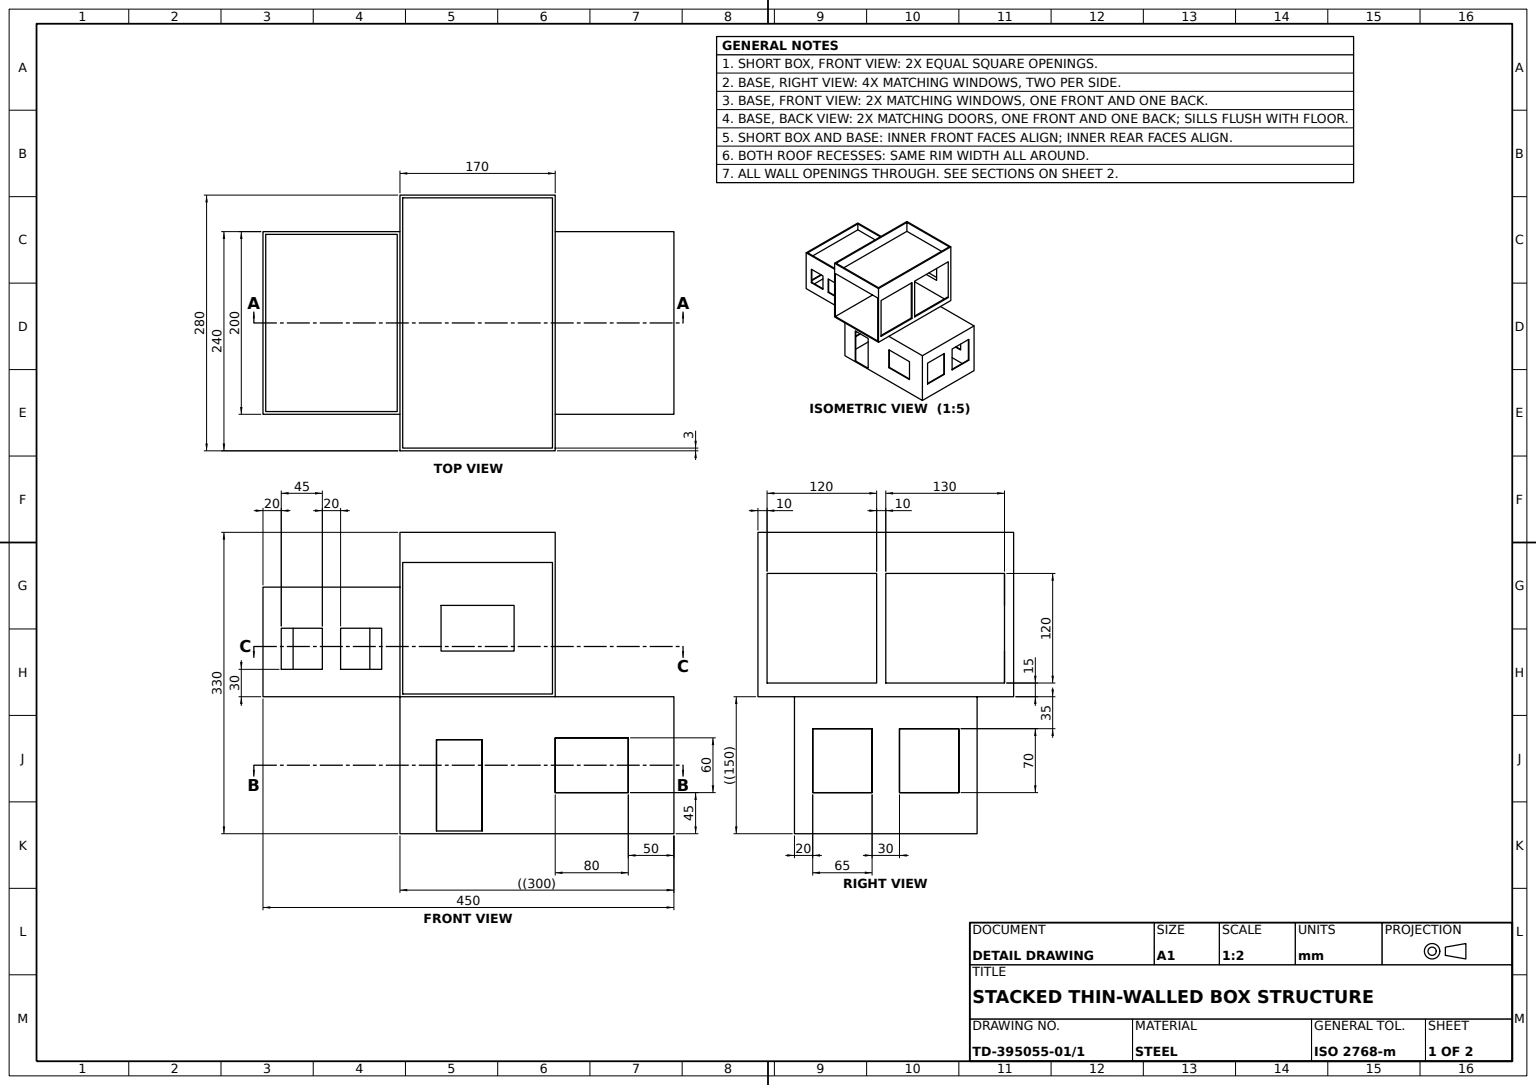
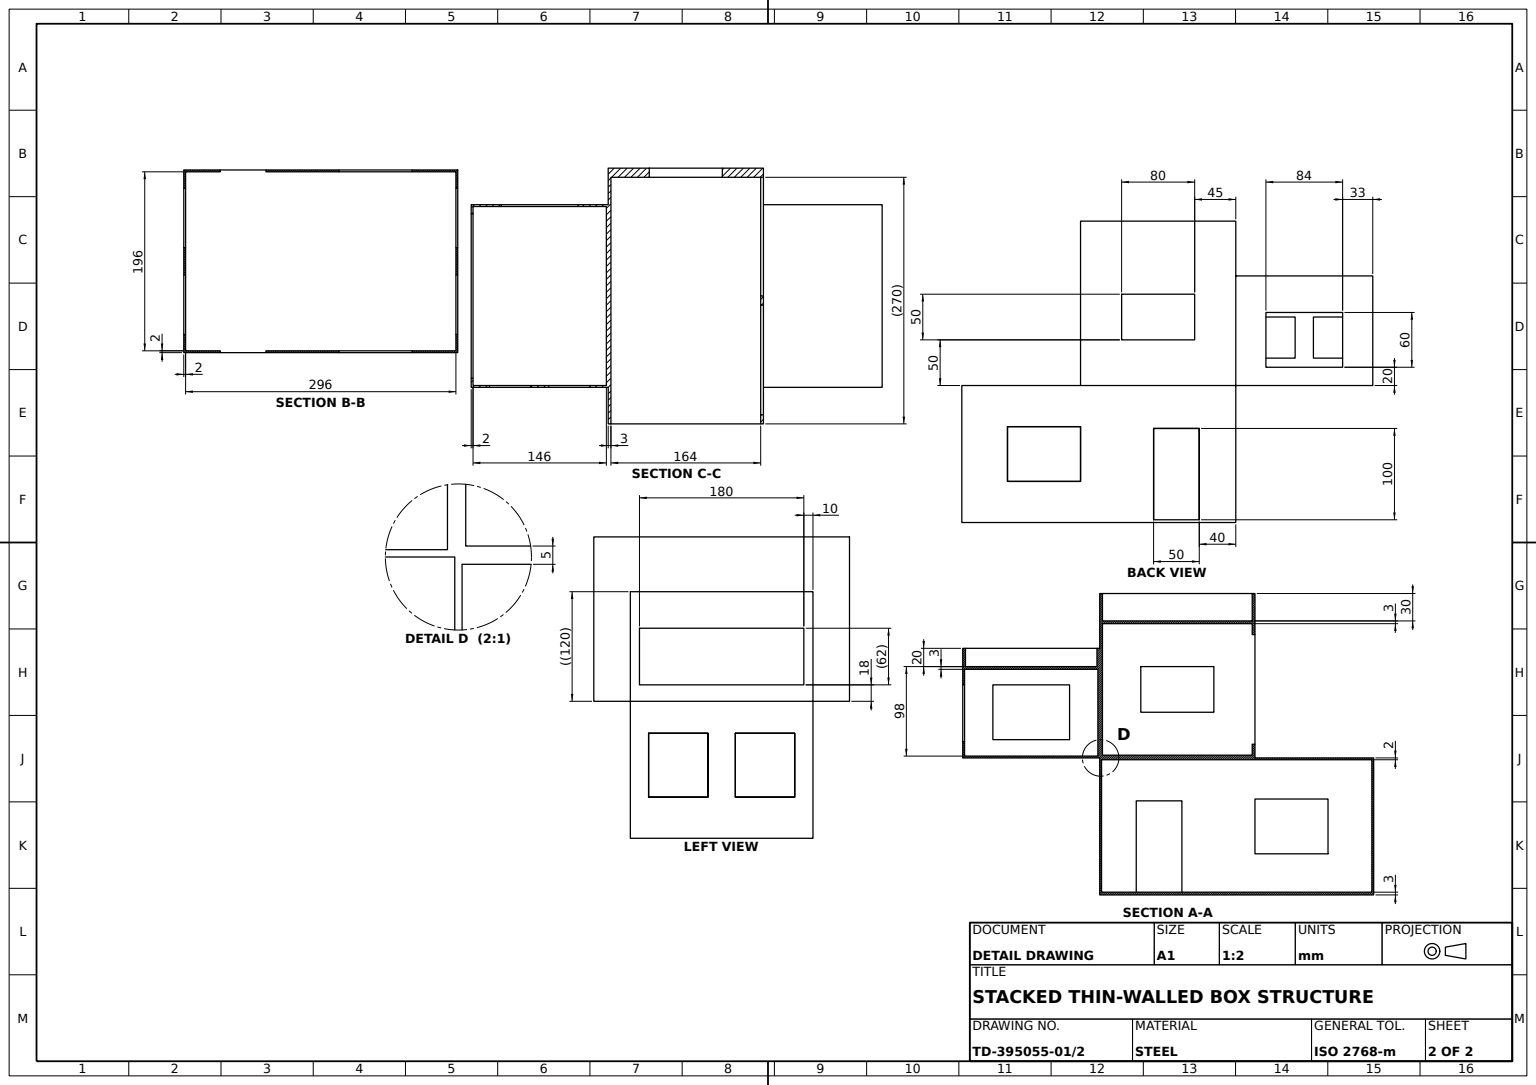
solid
v1 (-3,250,-3)
v2 (-3,250,-197)
e1 v1 v2 LINE
v3 (-3,270,-3)
e2 v1 v3 LINE
v4 (-3,270,-197)
e3 v4 v3 LINE
e4 v2 v4 LINE
face PLANE(AX(P(-3,0,0),D(1,0,0),D(0,0,-1))) rev [-e1 e2 -e3 -e4]
v5 (-150,270,0)
v6 (-150,150,0)
e5 v5 v6 LINE
v7 (-150,270,-200)
e6 v5 v7 LINE
v8 (-150,150,-200)
e7 v7 v8 LINE
e8 v8 v6 LINE
v9 (-150,168,-10)
v10 (-150,230,-10)
e9 v9 v10 LINE
v11 (-150,168,-190)
e10 v11 v9 LINE
v12 (-150,230,-190)
e11 v12 v11 LINE
e12 v10 v12 LINE
face PLANE(AX(P(-150,250,0),D(1,0,0),D(0,0,-1))) rev [-e5 e6 e7 e8] [-e9 -e10 -e11 -e12]
v13 (-65,180,-2)
v14 (-65,180,0)
e13 v13 v14 LINE
v15 (-20,180,0)
e14 v14 v15 LINE
v16 (-20,180,-2)
e15 v16 v15 LINE
e16 v13 v16 LINE
face PLANE(AX(P(-65,180,-23),D(0,-1,0),D(0,0,-1))) rev [e13 e14 -e15 -e16]
v17 (40,103,0)
v18 (40,3,0)
e17 v17 v18 LINE
v19 (90,103,0)
e18 v19 v17 LINE
v20 (90,3,0)
e19 v20 v19 LINE
e20 v18 v20 LINE
v21 (170,150,0)
v22 (300,150,0)
e21 v21 v22 LINE
v23 (0,150,0)
e22 v23 v21 LINE
v24 (0,0,0)
e23 v23 v24 LINE
v25 (300,0,0)
e24 v24 v25 LINE
e25 v22 v25 LINE
v26 (170,105,0)
v27 (170,45,0)
e26 v26 v27 LINE
v28 (250,105,0)
e27 v28 v26 LINE
v29 (250,45,0)
e28 v29 v28 LINE
e29 v27 v29 LINE
face PLANE(AX(P(0,150,0),D(0,0,-1),D(-1,0,0))) rev [-e17 -e18 -e19 -e20] [-e21 -e22 e23 e24 -e25] [-e26 -e27 -e28 -e29]
v30 (298,115,-85)
v31 (300,115,-85)
e30 v30 v31 LINE
v32 (298,45,-85)
e31 v32 v30 LINE
v33 (300,45,-85)
e32 v32 v33 LINE
e33 v33 v31 LINE
face PLANE(AX(P(-12,45,-85),D(0,0,-1),D(-1,0,0))) rev [-e30 -e31 e32 e33]
v34 (-65,225,-2)
e34 v34 v13 LINE
v35 (-65,225,0)
e35 v34 v35 LINE
e36 v35 v14 LINE
face PLANE(AX(P(-65,225,-23),D(-1,0,0),D(0,0,1))) rev [-e13 -e34 e35 e36]
v36 (3,300,-237)
v37 (3,300,37)
e37 v36 v37 LINE
v38 (3,330,-237)
e38 v38 v36 LINE
v39 (3,330,37)
e39 v39 v38 LINE
e40 v37 v39 LINE
face PLANE(AX(P(3,0,0),D(1,0,0),D(0,0,-1))) [-e37 -e38 -e39 -e40]
v40 (0,45,-20)
v41 (2,45,-20)
e41 v40 v41 LINE
v42 (2,45,-85)
e42 v42 v41 LINE
v43 (0,45,-85)
e43 v43 v42 LINE
e44 v40 v43 LINE
face PLANE(AX(P(-12,45,-20),D(0,-1,0),D(0,0,-1))) rev [e41 -e42 -e43 -e44]
v44 (167,300,-237)
e45 v44 v36 LINE
v45 (167,330,-237)
e46 v44 v45 LINE
e47 v38 v45 LINE
face PLANE(AX(P(0,0,-237),D(0,0,1),D(1,0,0))) [-e45 e46 -e47 e38]
v46 (-20,225,0)
e48 v15 v46 LINE
v47 (-20,225,-2)
e49 v47 v46 LINE
e50 v16 v47 LINE
face PLANE(AX(P(-20,225,-23),D(1,0,0),D(0,1,0))) rev [e15 e48 -e49 -e50]
v48 (40,3,-2)
v49 (40,103,-2)
e51 v48 v49 LINE
e52 v49 v17 LINE
e53 v48 v18 LINE
face PLANE(AX(P(40,3,-210),D(-1,0,0),D(0,0,1))) rev [e51 e52 e17 -e53]
v50 (-148,152,-198)
v51 (-148,247,-198)
e54 v50 v51 LINE
v52 (-2,152,-198)
e55 v52 v50 LINE
v53 (-2,247,-198)
e56 v52 v53 LINE
e57 v51 v53 LINE
v54 (-117,170,-198)
v55 (-117,230,-198)
e58 v54 v55 LINE
v56 (-33,230,-198)
e59 v55 v56 LINE
v57 (-33,170,-198)
e60 v56 v57 LINE
e61 v57 v54 LINE
face PLANE(AX(P(-148,152,-198),D(0,0,-1),D(-1,0,0))) rev [-e54 -e55 e56 -e57] [e58 e59 e60 e61]
v58 (-85,225,-2)
v59 (-85,225,0)
e62 v58 v59 LINE
v60 (-130,225,0)
e63 v59 v60 LINE
v61 (-130,225,-2)
e64 v61 v60 LINE
e65 v58 v61 LINE
face PLANE(AX(P(-130,225,-23),D(0,1,0),D(0,0,1))) rev [e62 e63 -e64 -e65]
v62 (45,200,-230)
v63 (45,250,-230)
e66 v62 v63 LINE
v64 (45,200,-240)
e67 v62 v64 LINE
v65 (45,250,-240)
e68 v64 v65 LINE
e69 v63 v65 LINE
face PLANE(AX(P(45,250,-140),D(-1,0,0),D(0,0,1))) rev [-e66 e67 e68 -e69]
v66 (170,45,-2)
v67 (250,45,-2)
e70 v66 v67 LINE
e71 v66 v27 LINE
e72 v67 v29 LINE
face PLANE(AX(P(170,45,-312),D(0,-1,0),D(0,0,-1))) rev [-e70 e71 e29 -e72]
v68 (125,200,-230)
e73 v68 v62 LINE
v69 (125,250,-230)
e74 v63 v69 LINE
e75 v69 v68 LINE
v70 (3,153,-230)
v71 (167,153,-230)
e76 v70 v71 LINE
v72 (167,165,-230)
e77 v71 v72 LINE
v73 (170,165,-230)
e78 v72 v73 LINE
v74 (170,285,-230)
e79 v73 v74 LINE
v75 (167,285,-230)
e80 v75 v74 LINE
v76 (167,297,-230)
e81 v75 v76 LINE
v77 (3,297,-230)
e82 v76 v77 LINE
e83 v77 v70 LINE
face PLANE(AX(P(0,0,-230),D(0,0,-1),D(-1,0,0))) rev [e73 e66 e74 e75] [e76 e77 e78 e79 -e80 e81 e82 e83]
v78 (-148,152,-2)
e84 v50 v78 LINE
v79 (-2,152,-2)
e85 v78 v79 LINE
e86 v79 v52 LINE
face PLANE(AX(P(0,152,0),D(0,1,0),D(0,0,1))) [e84 e85 e86 e55]
v80 (167,165,-100)
e87 v80 v72 LINE
v81 (170,165,-100)
e88 v80 v81 LINE
e89 v81 v73 LINE
face PLANE(AX(P(70,165,-100),D(0,-1,0),D(0,0,-1))) rev [-e78 -e87 e88 e89]
v82 (3,153,40)
e90 v70 v82 LINE
v83 (3,297,40)
e91 v77 v83 LINE
e92 v83 v82 LINE
face PLANE(AX(P(3,153,-230),D(-1,0,0),D(0,0,1))) rev [-e90 -e83 e91 e92]
v84 (-85,180,-2)
e93 v84 v58 LINE
v85 (-130,180,-2)
e94 v61 v85 LINE
e95 v85 v84 LINE
v86 (-2,247,-2)
v87 (-148,247,-2)
e96 v86 v87 LINE
e97 v79 v86 LINE
e98 v78 v87 LINE
e99 v47 v34 LINE
face PLANE(AX(P(-148,152,-2),D(0,0,1),D(1,0,0))) rev [e93 e65 e94 e95] [-e96 -e97 -e85 e98] [e16 e50 e99 e34]
v88 (0,150,-200)
e100 v23 v88 LINE
v89 (0,0,-200)
e101 v88 v89 LINE
e102 v89 v24 LINE
v90 (0,115,-85)
v91 (0,115,-20)
e103 v90 v91 LINE
e104 v91 v40 LINE
e105 v43 v90 LINE
v92 (0,115,-180)
v93 (0,115,-115)
e106 v92 v93 LINE
v94 (0,45,-115)
e107 v93 v94 LINE
v95 (0,45,-180)
e108 v94 v95 LINE
e109 v95 v92 LINE
face PLANE(AX(P(0,150,0),D(1,0,0),D(0,0,-1))) rev [-e23 e100 e101 e102] [e103 e104 e44 e105] [e106 e107 e108 e109]
v96 (-147,250,-197)
e110 v2 v96 LINE
v97 (-147,270,-197)
e111 v97 v4 LINE
e112 v97 v96 LINE
face PLANE(AX(P(0,0,-197),D(0,0,1),D(1,0,0))) [-e110 e4 -e111 e112]
v98 (167,300,37)
e113 v37 v98 LINE
e114 v98 v44 LINE
face PLANE(AX(P(0,300,40),D(0,-1,0),D(0,0,-1))) rev [e113 e114 e45 e37]
v99 (300,0,-200)
e115 v99 v89 LINE
e116 v25 v99 LINE
face PLANE(AX(P(0,0,0),D(0,-1,0),D(0,0,-1))) [-e102 -e115 -e116 -e24]
v100 (-148,230,-10)
e117 v100 v10 LINE
v101 (-148,168,-10)
e118 v101 v100 LINE
e119 v101 v9 LINE
face PLANE(AX(P(-127,168,-10),D(0,0,1),D(1,0,0))) rev [-e117 -e118 e119 e9]
v102 (2,148,-2)
v103 (2,148,-198)
e120 v102 v103 LINE
v104 (298,148,-198)
e121 v103 v104 LINE
v105 (298,148,-2)
e122 v104 v105 LINE
e123 v105 v102 LINE
face PLANE(AX(P(0,148,0),D(0,1,0),D(0,0,1))) rev [e120 e121 e122 e123]
v106 (167,330,37)
e124 v45 v106 LINE
e125 v98 v106 LINE
face PLANE(AX(P(167,0,0),D(1,0,0),D(0,0,-1))) rev [-e124 -e46 -e114 e125]
v107 (300,150,-200)
e126 v22 v107 LINE
v108 (170,150,-200)
e127 v107 v108 LINE
e128 v21 v108 LINE
face PLANE(AX(P(0,150,0),D(0,-1,0),D(0,0,-1))) rev [e21 e126 e127 -e128]
v109 (298,115,-115)
v110 (300,115,-115)
e129 v109 v110 LINE
v111 (298,115,-180)
e130 v111 v109 LINE
v112 (300,115,-180)
e131 v111 v112 LINE
e132 v112 v110 LINE
face PLANE(AX(P(-12,115,-115),D(0,1,0),D(0,0,1))) rev [-e129 -e130 e131 e132]
v113 (298,45,-20)
v114 (300,45,-20)
e133 v113 v114 LINE
e134 v114 v33 LINE
e135 v113 v32 LINE
face PLANE(AX(P(-12,45,-20),D(0,-1,0),D(0,0,-1))) rev [e133 e134 -e32 -e135]
v115 (167,285,-100)
e136 v75 v115 LINE
v116 (170,285,-100)
e137 v74 v116 LINE
e138 v115 v116 LINE
face PLANE(AX(P(70,285,-100),D(0,1,0),D(0,0,1))) rev [-e136 e80 e137 -e138]
v117 (2,45,-180)
v118 (2,45,-115)
e139 v117 v118 LINE
e140 v95 v117 LINE
e141 v94 v118 LINE
face PLANE(AX(P(-12,45,-115),D(0,-1,0),D(0,0,-1))) rev [-e139 -e140 -e108 e141]
e142 v53 v86 LINE
face PLANE(AX(P(-2,152,-198),D(1,0,0),D(0,0,-1))) rev [-e86 e97 -e142 -e56]
v119 (-148,168,-190)
e143 v119 v101 LINE
v120 (-148,230,-190)
e144 v100 v120 LINE
e145 v120 v119 LINE
e146 v87 v51 LINE
face PLANE(AX(P(-148,152,-198),D(-1,0,0),D(0,0,1))) rev [e143 e118 e144 e145] [e54 -e146 -e98 -e84]
v121 (90,103,-2)
e147 v121 v19 LINE
v122 (90,3,-2)
e148 v121 v122 LINE
e149 v122 v20 LINE
face PLANE(AX(P(90,3,-210),D(1,0,0),D(0,0,-1))) rev [-e147 e148 e149 e19]
v123 (-147,270,-3)
e150 v3 v123 LINE
e151 v123 v97 LINE
v124 (0,270,0)
e152 v124 v5 LINE
v125 (0,270,-200)
e153 v124 v125 LINE
e154 v125 v7 LINE
face PLANE(AX(P(-147,270,-200),D(0,1,0),D(0,0,1))) [e111 e3 e150 e151] [-e6 -e152 e153 e154]
v126 (0,150,40)
e155 v126 v23 LINE
v127 (170,150,40)
e156 v127 v21 LINE
e157 v126 v127 LINE
face PLANE(AX(P(0,150,40),D(0,1,0),D(0,0,1))) rev [e155 e22 -e156 -e157]
v128 (170,165,-90)
v129 (170,285,-90)
e158 v128 v129 LINE
v130 (167,285,-90)
e159 v130 v129 LINE
v131 (167,165,-90)
e160 v131 v130 LINE
e161 v131 v128 LINE
face PLANE(AX(P(70,165,-90),D(0,0,-1),D(-1,0,0))) rev [e158 -e159 -e160 e161]
v132 (167,297,40)
e162 v76 v132 LINE
e163 v132 v83 LINE
face PLANE(AX(P(3,297,-230),D(0,1,0),D(0,0,1))) rev [e162 e163 -e91 -e82]
v133 (125,250,-240)
e164 v65 v133 LINE
e165 v69 v133 LINE
face PLANE(AX(P(125,250,-140),D(0,1,0),D(0,0,1))) rev [e164 -e165 -e74 e69]
e166 v108 v88 LINE
e167 v107 v99 LINE
v134 (90,103,-200)
v135 (40,103,-200)
e168 v134 v135 LINE
v136 (40,3,-200)
e169 v135 v136 LINE
v137 (90,3,-200)
e170 v136 v137 LINE
e171 v137 v134 LINE
v138 (170,45,-200)
v139 (250,45,-200)
e172 v138 v139 LINE
v140 (250,105,-200)
e173 v139 v140 LINE
v141 (170,105,-200)
e174 v140 v141 LINE
e175 v141 v138 LINE
face PLANE(AX(P(0,150,-200),D(0,0,1),D(1,0,0))) rev [e115 -e101 -e166 -e127 e167] [e168 e169 e170 e171] [e172 e173 e174 e175]
e176 v119 v11 LINE
face PLANE(AX(P(-127,168,-190),D(0,-1,0),D(0,0,-1))) rev [e10 -e119 -e143 e176]
v142 (170,330,40)
e177 v127 v142 LINE
v143 (0,330,40)
e178 v143 v142 LINE
e179 v143 v126 LINE
v144 (167,153,40)
e180 v82 v144 LINE
e181 v144 v132 LINE
face PLANE(AX(P(0,0,40),D(0,0,-1),D(-1,0,0))) rev [e177 -e178 e179 e157] [-e180 -e92 -e163 -e181]
e182 v120 v12 LINE
face PLANE(AX(P(-127,168,-190),D(0,0,-1),D(-1,0,0))) rev [e182 e11 -e176 -e145]
v145 (2,115,-115)
e183 v118 v145 LINE
v146 (2,115,-180)
e184 v145 v146 LINE
e185 v146 v117 LINE
v147 (2,3,-2)
e186 v147 v102 LINE
v148 (2,3,-198)
e187 v148 v147 LINE
e188 v148 v103 LINE
v149 (2,115,-20)
e189 v41 v149 LINE
v150 (2,115,-85)
e190 v149 v150 LINE
e191 v150 v42 LINE
face PLANE(AX(P(2,-352.009859,-198),D(-1,0,0),D(0,0,1))) rev [e183 e184 e185 e139] [-e120 -e186 -e187 e188] [e42 e189 e190 e191]
v151 (298,115,-20)
e192 v30 v151 LINE
v152 (300,115,-20)
e193 v31 v152 LINE
e194 v151 v152 LINE
face PLANE(AX(P(-12,115,-20),D(0,1,0),D(0,0,1))) rev [-e192 e30 e193 -e194]
e195 v46 v35 LINE
face PLANE(AX(P(-65,225,-23),D(0,1,0),D(0,0,1))) rev [-e35 -e99 e49 e195]
v153 (298,45,-115)
v154 (298,45,-180)
e196 v153 v154 LINE
v155 (300,45,-115)
e197 v153 v155 LINE
v156 (300,45,-180)
e198 v155 v156 LINE
e199 v154 v156 LINE
face PLANE(AX(P(-12,45,-115),D(0,-1,0),D(0,0,-1))) rev [-e196 e197 e198 -e199]
e200 v116 v81 LINE
v157 (170,285,30)
e201 v129 v157 LINE
v158 (170,165,30)
e202 v158 v128 LINE
e203 v157 v158 LINE
v159 (170,150,-240)
e204 v108 v159 LINE
v160 (170,330,-240)
e205 v159 v160 LINE
e206 v142 v160 LINE
face PLANE(AX(P(170,150,40),D(-1,0,0),D(0,0,1))) rev [-e79 -e89 -e200 -e137] [-e201 -e158 -e202 -e203] [e156 e128 e204 e205 -e206 -e177]
v161 (125,200,-240)
e207 v68 v161 LINE
e208 v133 v161 LINE
face PLANE(AX(P(125,250,-140),D(1,0,0),D(0,0,-1))) rev [-e207 -e75 e165 e208]
e209 v90 v150 LINE
face PLANE(AX(P(-12,45,-85),D(0,0,-1),D(-1,0,0))) rev [-e105 e43 -e191 -e209]
e210 v71 v144 LINE
face PLANE(AX(P(3,153,-230),D(0,-1,0),D(0,0,-1))) rev [-e76 e90 e180 -e210]
v162 (0,150,-240)
e211 v88 v162 LINE
e212 v162 v159 LINE
face PLANE(AX(P(0,150,40),D(0,1,0),D(0,0,1))) rev [e211 e212 -e204 e166]
e213 v154 v111 LINE
e214 v156 v112 LINE
face PLANE(AX(P(-12,45,-180),D(0,0,-1),D(-1,0,0))) rev [-e131 -e213 e199 e214]
face PLANE(AX(P(0,247,0),D(0,1,0),D(0,0,1))) rev [e146 e57 e142 e96]
v163 (-147,250,-3)
e215 v163 v1 LINE
e216 v123 v163 LINE
face PLANE(AX(P(0,0,-3),D(0,0,1),D(1,0,0))) rev [-e2 -e215 -e216 -e150]
v164 (298,3,-2)
e217 v164 v105 LINE
e218 v122 v164 LINE
e219 v49 v121 LINE
e220 v147 v48 LINE
v165 (250,105,-2)
e221 v67 v165 LINE
v166 (170,105,-2)
e222 v165 v166 LINE
e223 v166 v66 LINE
face PLANE(AX(P(2,-352.009859,-2),D(0,0,1),D(1,0,0))) rev [-e123 -e217 -e218 -e148 -e219 -e51 -e220 e186] [e221 e222 e223 e70]
v167 (-33,230,-200)
v168 (-33,170,-200)
e224 v167 v168 LINE
e225 v57 v168 LINE
e226 v56 v167 LINE
face PLANE(AX(P(-33,170,-177),D(1,0,0),D(0,0,-1))) rev [e224 -e225 -e60 e226]
e227 v166 v26 LINE
face PLANE(AX(P(170,105,-312),D(-1,0,0),D(0,0,1))) rev [e227 e26 -e71 -e223]
v169 (250,105,-198)
e228 v140 v169 LINE
v170 (170,105,-198)
e229 v170 v169 LINE
e230 v141 v170 LINE
face PLANE(AX(P(170,105,-312),D(0,1,0),D(0,0,1))) rev [-e174 e228 -e229 -e230]
e231 v91 v149 LINE
face PLANE(AX(P(-12,45,-20),D(0,0,1),D(0,-1,0))) rev [-e189 -e41 -e104 e231]
e232 v152 v114 LINE
e233 v151 v113 LINE
face PLANE(AX(P(-12,45,-20),D(0,0,1),D(0,-1,0))) rev [e194 e232 -e133 -e233]
v171 (170,45,-198)
e234 v171 v170 LINE
e235 v138 v171 LINE
face PLANE(AX(P(170,105,-312),D(-1,0,0),D(0,0,1))) rev [-e234 -e235 -e175 e230]
v172 (250,45,-198)
e236 v139 v172 LINE
e237 v169 v172 LINE
face PLANE(AX(P(250,105,-312),D(1,0,0),D(0,0,-1))) rev [e236 -e237 -e228 -e173]
e238 v109 v153 LINE
v173 (298,3,-198)
e239 v173 v104 LINE
e240 v164 v173 LINE
face PLANE(AX(P(298,-352.009859,-198),D(1,0,0),D(0,0,-1))) rev [e130 e238 e196 e213] [e192 e233 e135 e31] [-e122 -e239 -e240 e217]
v174 (-117,170,-200)
e241 v168 v174 LINE
e242 v54 v174 LINE
face PLANE(AX(P(-117,170,-177),D(0,-1,0),D(0,0,-1))) rev [-e61 e225 e241 -e242]
e243 v125 v88 LINE
e244 v88 v8 LINE
v175 (-117,230,-200)
e245 v175 v167 LINE
e246 v174 v175 LINE
face PLANE(AX(P(0,250,-200),D(0,0,1),D(1,0,0))) rev [-e7 -e154 e243 e244] [-e241 -e224 -e245 -e246]
e247 v110 v155 LINE
face PLANE(AX(P(-12,45,-115),D(0,0,1),D(1,0,0))) rev [-e238 e129 e247 -e197]
e248 v92 v146 LINE
face PLANE(AX(P(-12,45,-180),D(0,0,-1),D(-1,0,0))) rev [-e185 -e248 -e109 e140]
v176 (167,165,30)
e249 v176 v131 LINE
e250 v176 v158 LINE
face PLANE(AX(P(70,165,30),D(0,-1,0),D(0,0,-1))) rev [-e249 e250 e202 -e161]
v177 (-130,180,0)
e251 v60 v177 LINE
e252 v85 v177 LINE
face PLANE(AX(P(-130,225,-23),D(-1,0,0),D(0,-1,0))) rev [-e94 e64 e251 -e252]
e253 v161 v64 LINE
face PLANE(AX(P(125,200,-140),D(0,-1,0),D(0,0,-1))) rev [-e73 e207 e253 -e67]
face PLANE(AX(P(-12,115,-20),D(0,1,0),D(0,0,1))) rev [-e231 -e103 e209 -e190]
e254 v93 v145 LINE
face PLANE(AX(P(-12,115,-115),D(0,1,0),D(0,0,1))) rev [-e184 -e254 -e106 e248]
e255 v115 v80 LINE
face PLANE(AX(P(70,285,-100),D(0,0,1),D(0,-1,0))) rev [-e255 e138 e200 -e88]
v178 (0,330,-240)
e256 v143 v178 LINE
e257 v178 v162 LINE
e258 v124 v23 LINE
face PLANE(AX(P(0,150,0),D(1,0,0),D(0,0,-1))) rev [e256 e257 -e211 -e243 -e153 e258 -e155 -e179]
face PLANE(AX(P(40,103,-210),D(0,1,0),D(0,0,1))) rev [-e52 e219 e147 e18]
v179 (167,285,30)
e259 v179 v176 LINE
e260 v179 v157 LINE
face PLANE(AX(P(70,165,30),D(0,0,1),D(0,-1,0))) rev [e203 -e250 -e259 e260]
e261 v6 v23 LINE
face PLANE(AX(P(0,150,0),D(0,1,0),D(0,0,1))) rev [-e8 -e244 -e100 -e261]
e262 v96 v163 LINE
face PLANE(AX(P(0,250,0),D(0,1,0),D(0,0,1))) [e215 e1 e110 e262]
v180 (-85,180,0)
e263 v84 v180 LINE
e264 v180 v59 LINE
face PLANE(AX(P(-85,225,-23),D(1,0,0),D(0,0,-1))) rev [-e93 e263 e264 -e62]
v181 (40,3,-198)
e265 v181 v148 LINE
v182 (40,103,-198)
e266 v182 v181 LINE
v183 (90,103,-198)
e267 v183 v182 LINE
v184 (90,3,-198)
e268 v184 v183 LINE
e269 v173 v184 LINE
e270 v172 v171 LINE
face PLANE(AX(P(2,-352.009859,-198),D(0,0,-1),D(-1,0,0))) rev [-e188 -e265 -e266 -e267 -e268 -e269 e239 -e121] [e270 e234 e229 e237]
e271 v130 v179 LINE
face PLANE(AX(P(167,153,-230),D(1,0,0),D(0,0,-1))) rev [-e77 e210 e181 -e162 -e81 e136 e255 e87] [e160 e271 e259 e249]
e272 v55 v175 LINE
face PLANE(AX(P(-117,230,-177),D(0,1,0),D(0,0,1))) rev [e245 -e226 -e59 e272]
face PLANE(AX(P(-147,0,0),D(1,0,0),D(0,0,-1))) [-e151 e216 -e262 -e112]
e273 v177 v180 LINE
face PLANE(AX(P(0,250,0),D(0,0,-1),D(-1,0,0))) rev [e152 e5 e261 -e258] [-e273 -e251 -e63 -e264] [-e14 -e36 -e195 -e48]
e274 v136 v181 LINE
e275 v135 v182 LINE
face PLANE(AX(P(40,3,-210),D(-1,0,0),D(0,0,1))) rev [e266 -e274 -e169 e275]
e276 v165 v28 LINE
face PLANE(AX(P(250,105,-312),D(1,0,0),D(0,0,-1))) rev [-e221 e72 e28 -e276]
e277 v137 v184 LINE
face PLANE(AX(P(40,3,-210),D(0,-1,0),D(0,0,-1))) rev [e218 e240 e269 -e277 -e170 e274 e265 e187 e220 e53 e20 -e149]
face PLANE(AX(P(-127,230,-190),D(0,1,0),D(0,0,1))) rev [e12 -e182 -e144 e117]
face PLANE(AX(P(-117,170,-177),D(-1,0,0),D(0,0,1))) rev [e242 e246 -e272 -e58]
e278 v134 v183 LINE
face PLANE(AX(P(90,3,-210),D(1,0,0),D(0,0,-1))) rev [e277 e268 -e278 -e171]
face PLANE(AX(P(170,105,-312),D(0,1,0),D(0,0,1))) rev [-e222 e276 e27 -e227]
face PLANE(AX(P(300,150,0),D(-1,0,0),D(0,0,1))) rev [-e33 -e134 -e232 -e193] [-e167 -e126 e25 e116] [-e214 -e198 -e247 -e132]
face PLANE(AX(P(70,285,30),D(0,1,0),D(0,0,1))) rev [e159 e201 -e260 -e271]
e279 v106 v39 LINE
e280 v178 v160 LINE
face PLANE(AX(P(170,330,-237),D(0,1,0),D(0,0,1))) [e124 e279 e39 e47] [-e256 e178 e206 -e280]
face PLANE(AX(P(170,45,-312),D(0,-1,0),D(0,0,-1))) rev [-e172 e235 -e270 -e236]
face PLANE(AX(P(0,0,-240),D(0,0,-1),D(-1,0,0))) [-e205 -e212 -e257 e280] [-e68 -e253 -e208 -e164]
face PLANE(AX(P(-130,180,-23),D(0,-1,0),D(0,0,-1))) rev [e273 -e263 -e95 e252]
face PLANE(AX(P(0,0,37),D(0,0,-1),D(-1,0,0))) [e40 -e279 -e125 -e113]
face PLANE(AX(P(40,103,-210),D(0,1,0),D(0,0,1))) rev [e278 e267 -e275 -e168]
face PLANE(AX(P(-12,45,-115),D(0,0,1),D(1,0,0))) rev [-e141 -e107 e254 -e183]
